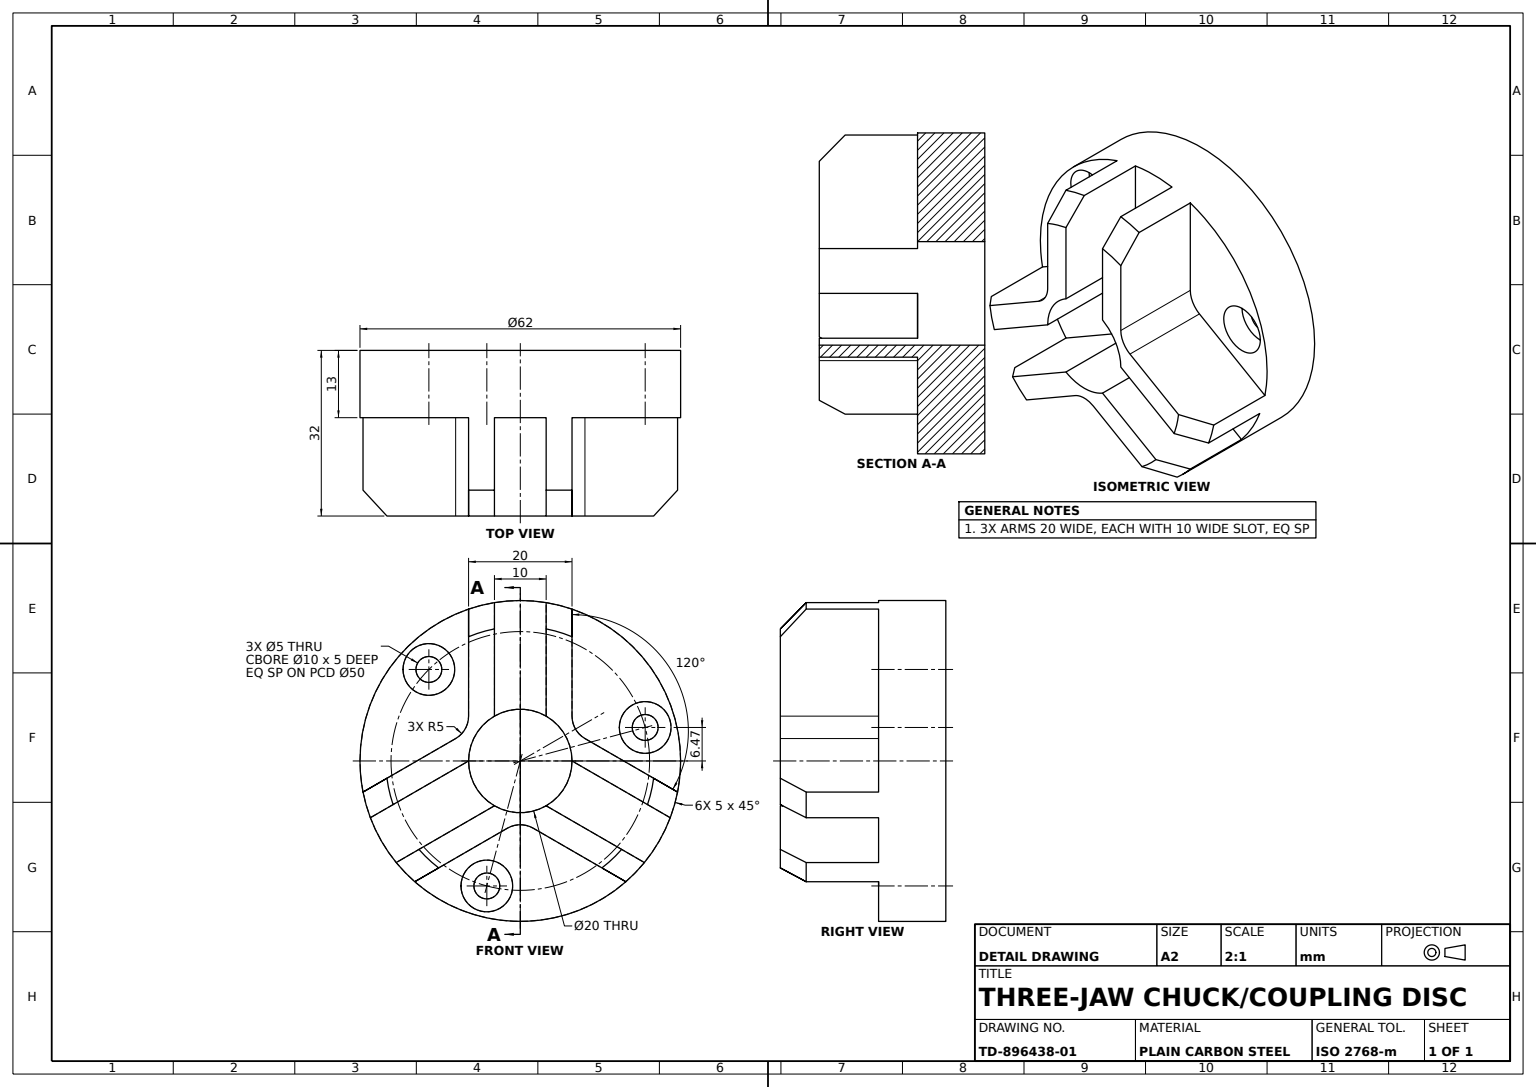
ISO-10303-21;
HEADER;
FILE_DESCRIPTION((''),'2;1');
FILE_NAME('','',(''),(''),'','','');
FILE_SCHEMA(('AUTOMOTIVE_DESIGN'));
ENDSEC;
DATA;
#1=APPLICATION_CONTEXT('');
#2=PRODUCT_CONTEXT('',#1,'mechanical');
#3=PRODUCT('','','',(#2));
#4=PRODUCT_DEFINITION_FORMATION('','',#3);
#5=PRODUCT_DEFINITION_CONTEXT('',#1,'design');
#6=PRODUCT_DEFINITION('','',#4,#5);
#7=PRODUCT_DEFINITION_SHAPE('','',#6);
#8=(LENGTH_UNIT()NAMED_UNIT(*)SI_UNIT(.MILLI.,.METRE.));
#9=(NAMED_UNIT(*)PLANE_ANGLE_UNIT()SI_UNIT($,.RADIAN.));
#10=(NAMED_UNIT(*)SI_UNIT($,.STERADIAN.)SOLID_ANGLE_UNIT());
#11=UNCERTAINTY_MEASURE_WITH_UNIT(LENGTH_MEASURE(1.E-05),#8,'distance_accuracy_value','');
#12=(GEOMETRIC_REPRESENTATION_CONTEXT(3)GLOBAL_UNCERTAINTY_ASSIGNED_CONTEXT((#11))GLOBAL_UNIT_ASSIGNED_CONTEXT((#8,#9,#10))REPRESENTATION_CONTEXT('',''));
#13=CARTESIAN_POINT('',(25.78461,-3.339746,32.));
#14=VERTEX_POINT('',#13);
#15=CARTESIAN_POINT('',(30.411612,-6.011147,27.));
#16=VERTEX_POINT('',#15);
#17=CARTESIAN_POINT('',(27.336826,-4.235919,30.345527));
#18=CARTESIAN_POINT('',(28.87747,-5.12541,28.676775));
#19=B_SPLINE_CURVE_WITH_KNOTS('',3,(#13,#17,#18,#15),.UNSPECIFIED.,.F.,.F.,(4,4),(0.,0.007317481),.UNSPECIFIED.);
#20=EDGE_CURVE('',#14,#16,#19,.T.);
#21=ORIENTED_EDGE('',*,*,#20,.T.);
#22=CARTESIAN_POINT('',(30.411612,-6.011147,13.));
#23=VERTEX_POINT('',#22);
#24=CARTESIAN_POINT('',(30.411612,-6.011147,32.));
#25=DIRECTION('',(0.,0.,-1.));
#26=VECTOR('',#25,1000.);
#27=LINE('',#24,#26);
#28=EDGE_CURVE('',#16,#23,#27,.T.);
#29=ORIENTED_EDGE('',*,*,#28,.T.);
#30=CARTESIAN_POINT('',(12.5,4.330127,13.));
#31=VERTEX_POINT('',#30);
#32=CARTESIAN_POINT('',(5.,8.660254,13.));
#33=DIRECTION('',(0.866025404,-0.5,0.));
#34=VECTOR('',#33,1000.);
#35=LINE('',#32,#34);
#36=EDGE_CURVE('',#31,#23,#35,.T.);
#37=ORIENTED_EDGE('',*,*,#36,.F.);
#38=CARTESIAN_POINT('',(12.5,4.330127,32.));
#39=VERTEX_POINT('',#38);
#40=LINE('',#38,#26);
#41=EDGE_CURVE('',#39,#31,#40,.T.);
#42=ORIENTED_EDGE('',*,*,#41,.F.);
#43=CARTESIAN_POINT('',(5.,8.660254,32.));
#44=LINE('',#43,#34);
#45=EDGE_CURVE('',#39,#14,#44,.T.);
#46=ORIENTED_EDGE('',*,*,#45,.T.);
#47=EDGE_LOOP('',(#21,#29,#37,#42,#46));
#48=FACE_OUTER_BOUND('',#47,.T.);
#49=DIRECTION('',(0.5,0.866025404,0.));
#50=DIRECTION('',(-0.866025404,0.5,0.));
#51=AXIS2_PLACEMENT_3D('',#43,#49,#50);
#52=PLANE('',#51);
#53=ADVANCED_FACE('',(#48),#52,.T.);
#54=CARTESIAN_POINT('',(-5.,-8.660254,32.));
#55=VERTEX_POINT('',#54);
#56=CARTESIAN_POINT('',(-5.,-8.660254,13.));
#57=VERTEX_POINT('',#56);
#58=LINE('',#54,#26);
#59=EDGE_CURVE('',#55,#57,#58,.T.);
#60=ORIENTED_EDGE('',*,*,#59,.F.);
#61=CARTESIAN_POINT('',(5.,-8.660254,32.));
#62=VERTEX_POINT('',#61);
#63=CARTESIAN_POINT('',(0.,0.,32.));
#64=DIRECTION('',(1.,0.,0.));
#65=AXIS2_PLACEMENT_3D('',#63,#25,#64);
#66=CIRCLE('',#65,10.);
#67=EDGE_CURVE('',#62,#55,#66,.T.);
#68=ORIENTED_EDGE('',*,*,#67,.F.);
#69=CARTESIAN_POINT('',(5.,-8.660254,13.));
#70=VERTEX_POINT('',#69);
#71=LINE('',#61,#26);
#72=EDGE_CURVE('',#62,#70,#71,.T.);
#73=ORIENTED_EDGE('',*,*,#72,.T.);
#74=CARTESIAN_POINT('',(10.,0.,13.));
#75=VERTEX_POINT('',#74);
#76=CARTESIAN_POINT('',(0.,0.,13.));
#77=DIRECTION('',(0.,0.,1.));
#78=AXIS2_PLACEMENT_3D('',#76,#77,#64);
#79=CIRCLE('',#78,10.);
#80=EDGE_CURVE('',#70,#75,#79,.T.);
#81=ORIENTED_EDGE('',*,*,#80,.T.);
#82=CARTESIAN_POINT('',(10.,0.,0.));
#83=VERTEX_POINT('',#82);
#84=VECTOR('',#77,1000.);
#85=LINE('',#82,#84);
#86=EDGE_CURVE('',#83,#75,#85,.T.);
#87=ORIENTED_EDGE('',*,*,#86,.F.);
#88=CARTESIAN_POINT('',(-10.,0.,0.));
#89=VERTEX_POINT('',#88);
#90=CARTESIAN_POINT('',(0.,0.,0.));
#91=AXIS2_PLACEMENT_3D('',#90,#77,#64);
#92=CIRCLE('',#91,10.);
#93=EDGE_CURVE('',#89,#83,#92,.T.);
#94=ORIENTED_EDGE('',*,*,#93,.F.);
#95=CARTESIAN_POINT('',(-10.,0.,13.));
#96=VERTEX_POINT('',#95);
#97=LINE('',#88,#84);
#98=EDGE_CURVE('',#89,#96,#97,.T.);
#99=ORIENTED_EDGE('',*,*,#98,.T.);
#100=EDGE_CURVE('',#96,#57,#79,.T.);
#101=ORIENTED_EDGE('',*,*,#100,.T.);
#102=EDGE_LOOP('',(#60,#68,#73,#81,#87,#94,#99,#101));
#103=FACE_OUTER_BOUND('',#102,.T.);
#104=CYLINDRICAL_SURFACE('',#91,10.);
#105=ADVANCED_FACE('',(#103),#104,.F.);
#106=CARTESIAN_POINT('',(-5.,8.660254,13.));
#107=VERTEX_POINT('',#106);
#108=CARTESIAN_POINT('',(-5.,30.594117,13.));
#109=VERTEX_POINT('',#108);
#110=CARTESIAN_POINT('',(-5.,0.,13.));
#111=DIRECTION('',(0.,1.,0.));
#112=VECTOR('',#111,1000.);
#113=LINE('',#110,#112);
#114=EDGE_CURVE('',#107,#109,#113,.T.);
#115=ORIENTED_EDGE('',*,*,#114,.T.);
#116=CARTESIAN_POINT('',(-5.,30.594117,27.));
#117=VERTEX_POINT('',#116);
#118=CARTESIAN_POINT('',(-5.,30.594117,32.));
#119=LINE('',#118,#26);
#120=EDGE_CURVE('',#117,#109,#119,.T.);
#121=ORIENTED_EDGE('',*,*,#120,.F.);
#122=CARTESIAN_POINT('',(-5.,25.514702,32.));
#123=VERTEX_POINT('',#122);
#124=CARTESIAN_POINT('',(-5.,28.903127,28.66885));
#125=CARTESIAN_POINT('',(-5.,27.210409,30.335943));
#126=B_SPLINE_CURVE_WITH_KNOTS('',3,(#116,#124,#125,#122),.UNSPECIFIED.,.F.,.F.,(4,4),(0.,0.007127444),.UNSPECIFIED.);
#127=EDGE_CURVE('',#117,#123,#126,.T.);
#128=ORIENTED_EDGE('',*,*,#127,.T.);
#129=CARTESIAN_POINT('',(-5.,8.660254,32.));
#130=VERTEX_POINT('',#129);
#131=CARTESIAN_POINT('',(-5.,0.,32.));
#132=LINE('',#131,#112);
#133=EDGE_CURVE('',#130,#123,#132,.T.);
#134=ORIENTED_EDGE('',*,*,#133,.F.);
#135=LINE('',#129,#26);
#136=EDGE_CURVE('',#130,#107,#135,.T.);
#137=ORIENTED_EDGE('',*,*,#136,.T.);
#138=EDGE_LOOP('',(#115,#121,#128,#134,#137));
#139=FACE_OUTER_BOUND('',#138,.T.);
#140=DIRECTION('',(-1.,0.,0.));
#141=AXIS2_PLACEMENT_3D('',#131,#140,#77);
#142=PLANE('',#141);
#143=ADVANCED_FACE('',(#139),#142,.F.);
#144=CARTESIAN_POINT('',(5.,30.594117,13.));
#145=VERTEX_POINT('',#144);
#146=CIRCLE('',#78,31.);
#147=EDGE_CURVE('',#145,#109,#146,.T.);
#148=ORIENTED_EDGE('',*,*,#147,.T.);
#149=ORIENTED_EDGE('',*,*,#114,.F.);
#150=VERTEX_POINT('',#32);
#151=EDGE_CURVE('',#150,#107,#79,.T.);
#152=ORIENTED_EDGE('',*,*,#151,.F.);
#153=CARTESIAN_POINT('',(5.,0.,13.));
#154=LINE('',#153,#112);
#155=EDGE_CURVE('',#150,#145,#154,.T.);
#156=ORIENTED_EDGE('',*,*,#155,.T.);
#157=EDGE_LOOP('',(#148,#149,#152,#156));
#158=FACE_OUTER_BOUND('',#157,.T.);
#159=PLANE('',#78);
#160=ADVANCED_FACE('',(#158),#159,.T.);
#161=CARTESIAN_POINT('',(-28.995283,-10.966932,13.));
#162=VERTEX_POINT('',#161);
#163=CARTESIAN_POINT('',(-2.5,4.330127,13.));
#164=DIRECTION('',(-0.866025404,-0.5,0.));
#165=VECTOR('',#164,1000.);
#166=LINE('',#163,#165);
#167=EDGE_CURVE('',#96,#162,#166,.T.);
#168=ORIENTED_EDGE('',*,*,#167,.T.);
#169=CARTESIAN_POINT('',(-23.995283,-19.627186,13.));
#170=VERTEX_POINT('',#169);
#171=EDGE_CURVE('',#162,#170,#146,.T.);
#172=ORIENTED_EDGE('',*,*,#171,.T.);
#173=CARTESIAN_POINT('',(2.5,-4.330127,13.));
#174=LINE('',#173,#165);
#175=EDGE_CURVE('',#57,#170,#174,.T.);
#176=ORIENTED_EDGE('',*,*,#175,.F.);
#177=ORIENTED_EDGE('',*,*,#100,.F.);
#178=EDGE_LOOP('',(#168,#172,#176,#177));
#179=FACE_OUTER_BOUND('',#178,.T.);
#180=ADVANCED_FACE('',(#179),#159,.T.);
#181=CARTESIAN_POINT('',(-1.470476,-24.148146,13.));
#182=VERTEX_POINT('',#181);
#183=CARTESIAN_POINT('',(-11.470476,-24.148146,13.));
#184=VERTEX_POINT('',#183);
#185=CARTESIAN_POINT('',(-6.470476,-24.148146,13.));
#186=AXIS2_PLACEMENT_3D('',#185,#77,#64);
#187=CIRCLE('',#186,5.);
#188=EDGE_CURVE('',#182,#184,#187,.T.);
#189=ORIENTED_EDGE('',*,*,#188,.F.);
#190=EDGE_CURVE('',#184,#182,#187,.T.);
#191=ORIENTED_EDGE('',*,*,#190,.F.);
#192=EDGE_LOOP('',(#189,#191));
#193=FACE_BOUND('',#192,.T.);
#194=CARTESIAN_POINT('',(2.5,-12.990381,13.));
#195=VERTEX_POINT('',#194);
#196=CARTESIAN_POINT('',(-2.5,-12.990381,13.));
#197=VERTEX_POINT('',#196);
#198=CARTESIAN_POINT('',(0.,-17.320508,13.));
#199=AXIS2_PLACEMENT_3D('',#198,#77,#64);
#200=CIRCLE('',#199,5.);
#201=EDGE_CURVE('',#195,#197,#200,.T.);
#202=ORIENTED_EDGE('',*,*,#201,.T.);
#203=CARTESIAN_POINT('',(-20.411612,-23.331655,13.));
#204=VERTEX_POINT('',#203);
#205=LINE('',#69,#165);
#206=EDGE_CURVE('',#197,#204,#205,.T.);
#207=ORIENTED_EDGE('',*,*,#206,.T.);
#208=CARTESIAN_POINT('',(20.411612,-23.331655,13.));
#209=VERTEX_POINT('',#208);
#210=EDGE_CURVE('',#204,#209,#146,.T.);
#211=ORIENTED_EDGE('',*,*,#210,.T.);
#212=LINE('',#56,#34);
#213=EDGE_CURVE('',#195,#209,#212,.T.);
#214=ORIENTED_EDGE('',*,*,#213,.F.);
#215=EDGE_LOOP('',(#202,#207,#211,#214));
#216=FACE_OUTER_BOUND('',#215,.T.);
#217=ADVANCED_FACE('',(#193,#216),#159,.T.);
#218=CARTESIAN_POINT('',(26.648146,6.470476,0.));
#219=VERTEX_POINT('',#218);
#220=CARTESIAN_POINT('',(26.648146,6.470476,8.));
#221=VERTEX_POINT('',#220);
#222=LINE('',#218,#84);
#223=EDGE_CURVE('',#219,#221,#222,.T.);
#224=ORIENTED_EDGE('',*,*,#223,.T.);
#225=CARTESIAN_POINT('',(21.648146,6.470476,8.));
#226=VERTEX_POINT('',#225);
#227=CARTESIAN_POINT('',(24.148146,6.470476,8.));
#228=AXIS2_PLACEMENT_3D('',#227,#25,#64);
#229=CIRCLE('',#228,2.5);
#230=EDGE_CURVE('',#226,#221,#229,.T.);
#231=ORIENTED_EDGE('',*,*,#230,.F.);
#232=CARTESIAN_POINT('',(21.648146,6.470476,0.));
#233=VERTEX_POINT('',#232);
#234=LINE('',#232,#84);
#235=EDGE_CURVE('',#233,#226,#234,.T.);
#236=ORIENTED_EDGE('',*,*,#235,.F.);
#237=CARTESIAN_POINT('',(24.148146,6.470476,0.));
#238=DIRECTION('',(-0.5,0.866025404,0.));
#239=AXIS2_PLACEMENT_3D('',#237,#77,#238);
#240=CIRCLE('',#239,2.5);
#241=EDGE_CURVE('',#219,#233,#240,.T.);
#242=ORIENTED_EDGE('',*,*,#241,.F.);
#243=EDGE_LOOP('',(#224,#231,#236,#242));
#244=FACE_OUTER_BOUND('',#243,.T.);
#245=AXIS2_PLACEMENT_3D('',#237,#77,#64);
#246=CYLINDRICAL_SURFACE('',#245,2.5);
#247=ADVANCED_FACE('',(#244),#246,.F.);
#248=ORIENTED_EDGE('',*,*,#20,.F.);
#249=CARTESIAN_POINT('',(24.59638,-8.427224,32.));
#250=VERTEX_POINT('',#249);
#251=AXIS2_PLACEMENT_3D('',#63,#77,#64);
#252=CIRCLE('',#251,26.);
#253=EDGE_CURVE('',#250,#14,#252,.T.);
#254=ORIENTED_EDGE('',*,*,#253,.F.);
#255=CARTESIAN_POINT('',(28.995283,-10.966932,27.));
#256=VERTEX_POINT('',#255);
#257=CARTESIAN_POINT('',(27.530843,-10.121437,28.66885));
#258=CARTESIAN_POINT('',(26.064906,-9.275078,30.335943));
#259=B_SPLINE_CURVE_WITH_KNOTS('',3,(#255,#257,#258,#249),.UNSPECIFIED.,.F.,.F.,(4,4),(0.,0.007127444),.UNSPECIFIED.);
#260=EDGE_CURVE('',#256,#250,#259,.T.);
#261=ORIENTED_EDGE('',*,*,#260,.F.);
#262=CARTESIAN_POINT('',(0.,0.,27.));
#263=AXIS2_PLACEMENT_3D('',#262,#25,#64);
#264=CIRCLE('',#263,31.);
#265=EDGE_CURVE('',#16,#256,#264,.T.);
#266=ORIENTED_EDGE('',*,*,#265,.F.);
#267=EDGE_LOOP('',(#248,#254,#261,#266));
#268=FACE_OUTER_BOUND('',#267,.T.);
#269=AXIS2_PLACEMENT_3D('',#63,#25,#140);
#270=CONICAL_SURFACE('',#269,26.,0.785398163);
#271=ADVANCED_FACE('',(#268),#270,.T.);
#272=CARTESIAN_POINT('',(10.,29.342802,27.));
#273=VERTEX_POINT('',#272);
#274=CARTESIAN_POINT('',(10.,29.342802,13.));
#275=VERTEX_POINT('',#274);
#276=CARTESIAN_POINT('',(10.,29.342802,32.));
#277=LINE('',#276,#26);
#278=EDGE_CURVE('',#273,#275,#277,.T.);
#279=ORIENTED_EDGE('',*,*,#278,.F.);
#280=CARTESIAN_POINT('',(10.,24.,32.));
#281=VERTEX_POINT('',#280);
#282=CARTESIAN_POINT('',(10.,27.571327,28.676775));
#283=CARTESIAN_POINT('',(10.,25.792345,30.345527));
#284=B_SPLINE_CURVE_WITH_KNOTS('',3,(#272,#282,#283,#280),.UNSPECIFIED.,.F.,.F.,(4,4),(0.,0.007317481),.UNSPECIFIED.);
#285=EDGE_CURVE('',#273,#281,#284,.T.);
#286=ORIENTED_EDGE('',*,*,#285,.T.);
#287=CARTESIAN_POINT('',(10.,8.660254,32.));
#288=VERTEX_POINT('',#287);
#289=CARTESIAN_POINT('',(10.,0.,32.));
#290=LINE('',#289,#112);
#291=EDGE_CURVE('',#288,#281,#290,.T.);
#292=ORIENTED_EDGE('',*,*,#291,.F.);
#293=CARTESIAN_POINT('',(10.,8.660254,13.));
#294=VERTEX_POINT('',#293);
#295=LINE('',#287,#26);
#296=EDGE_CURVE('',#288,#294,#295,.T.);
#297=ORIENTED_EDGE('',*,*,#296,.T.);
#298=LINE('',#74,#112);
#299=EDGE_CURVE('',#294,#275,#298,.T.);
#300=ORIENTED_EDGE('',*,*,#299,.T.);
#301=EDGE_LOOP('',(#279,#286,#292,#297,#300));
#302=FACE_OUTER_BOUND('',#301,.T.);
#303=AXIS2_PLACEMENT_3D('',#289,#140,#77);
#304=PLANE('',#303);
#305=ADVANCED_FACE('',(#302),#304,.F.);
#306=CARTESIAN_POINT('',(-19.59638,-17.087478,32.));
#307=VERTEX_POINT('',#306);
#308=CARTESIAN_POINT('',(-15.78461,-20.660254,32.));
#309=VERTEX_POINT('',#308);
#310=EDGE_CURVE('',#307,#309,#252,.T.);
#311=ORIENTED_EDGE('',*,*,#310,.T.);
#312=CARTESIAN_POINT('',(-2.5,-12.990381,32.));
#313=VERTEX_POINT('',#312);
#314=LINE('',#61,#165);
#315=EDGE_CURVE('',#313,#309,#314,.T.);
#316=ORIENTED_EDGE('',*,*,#315,.F.);
#317=CARTESIAN_POINT('',(2.5,-12.990381,32.));
#318=VERTEX_POINT('',#317);
#319=CARTESIAN_POINT('',(0.,-17.320508,32.));
#320=AXIS2_PLACEMENT_3D('',#319,#77,#64);
#321=CIRCLE('',#320,5.);
#322=EDGE_CURVE('',#318,#313,#321,.T.);
#323=ORIENTED_EDGE('',*,*,#322,.F.);
#324=CARTESIAN_POINT('',(15.78461,-20.660254,32.));
#325=VERTEX_POINT('',#324);
#326=LINE('',#54,#34);
#327=EDGE_CURVE('',#318,#325,#326,.T.);
#328=ORIENTED_EDGE('',*,*,#327,.T.);
#329=CARTESIAN_POINT('',(19.59638,-17.087478,32.));
#330=VERTEX_POINT('',#329);
#331=EDGE_CURVE('',#325,#330,#252,.T.);
#332=ORIENTED_EDGE('',*,*,#331,.T.);
#333=CARTESIAN_POINT('',(-2.5,-4.330127,32.));
#334=LINE('',#333,#34);
#335=EDGE_CURVE('',#62,#330,#334,.T.);
#336=ORIENTED_EDGE('',*,*,#335,.F.);
#337=ORIENTED_EDGE('',*,*,#67,.T.);
#338=CARTESIAN_POINT('',(2.5,-4.330127,32.));
#339=LINE('',#338,#165);
#340=EDGE_CURVE('',#55,#307,#339,.T.);
#341=ORIENTED_EDGE('',*,*,#340,.T.);
#342=EDGE_LOOP('',(#311,#316,#323,#328,#332,#336,#337,#341));
#343=FACE_OUTER_BOUND('',#342,.T.);
#344=PLANE('',#251);
#345=ADVANCED_FACE('',(#343),#344,.T.);
#346=CARTESIAN_POINT('',(-8.970476,-24.148146,0.));
#347=VERTEX_POINT('',#346);
#348=CARTESIAN_POINT('',(-3.970476,-24.148146,0.));
#349=VERTEX_POINT('',#348);
#350=CARTESIAN_POINT('',(-6.470476,-24.148146,0.));
#351=AXIS2_PLACEMENT_3D('',#350,#77,#64);
#352=CIRCLE('',#351,2.5);
#353=EDGE_CURVE('',#347,#349,#352,.T.);
#354=ORIENTED_EDGE('',*,*,#353,.F.);
#355=CARTESIAN_POINT('',(-8.970476,-24.148146,8.));
#356=VERTEX_POINT('',#355);
#357=LINE('',#346,#84);
#358=EDGE_CURVE('',#347,#356,#357,.T.);
#359=ORIENTED_EDGE('',*,*,#358,.T.);
#360=CARTESIAN_POINT('',(-3.970476,-24.148146,8.));
#361=VERTEX_POINT('',#360);
#362=CARTESIAN_POINT('',(-6.470476,-24.148146,8.));
#363=AXIS2_PLACEMENT_3D('',#362,#25,#64);
#364=CIRCLE('',#363,2.5);
#365=EDGE_CURVE('',#361,#356,#364,.T.);
#366=ORIENTED_EDGE('',*,*,#365,.F.);
#367=LINE('',#348,#84);
#368=EDGE_CURVE('',#349,#361,#367,.T.);
#369=ORIENTED_EDGE('',*,*,#368,.F.);
#370=EDGE_LOOP('',(#354,#359,#366,#369));
#371=FACE_OUTER_BOUND('',#370,.T.);
#372=CYLINDRICAL_SURFACE('',#351,2.5);
#373=ADVANCED_FACE('',(#371),#372,.F.);
#374=CARTESIAN_POINT('',(23.995283,-19.627186,27.));
#375=VERTEX_POINT('',#374);
#376=CARTESIAN_POINT('',(20.411612,-23.331655,27.));
#377=VERTEX_POINT('',#376);
#378=EDGE_CURVE('',#375,#377,#264,.T.);
#379=ORIENTED_EDGE('',*,*,#378,.F.);
#380=CARTESIAN_POINT('',(21.064906,-17.935332,30.335943));
#381=CARTESIAN_POINT('',(22.530843,-18.781691,28.66885));
#382=B_SPLINE_CURVE_WITH_KNOTS('',3,(#329,#380,#381,#374),.UNSPECIFIED.,.F.,.F.,(4,4),(0.,0.007127444),.UNSPECIFIED.);
#383=EDGE_CURVE('',#330,#375,#382,.T.);
#384=ORIENTED_EDGE('',*,*,#383,.F.);
#385=ORIENTED_EDGE('',*,*,#331,.F.);
#386=CARTESIAN_POINT('',(18.87747,-22.445918,28.676775));
#387=CARTESIAN_POINT('',(17.336826,-21.556427,30.345527));
#388=B_SPLINE_CURVE_WITH_KNOTS('',3,(#376,#386,#387,#324),.UNSPECIFIED.,.F.,.F.,(4,4),(0.,0.007317481),.UNSPECIFIED.);
#389=EDGE_CURVE('',#377,#325,#388,.T.);
#390=ORIENTED_EDGE('',*,*,#389,.F.);
#391=EDGE_LOOP('',(#379,#384,#385,#390));
#392=FACE_OUTER_BOUND('',#391,.T.);
#393=ADVANCED_FACE('',(#392),#270,.T.);
#394=ORIENTED_EDGE('',*,*,#253,.T.);
#395=ORIENTED_EDGE('',*,*,#45,.F.);
#396=CARTESIAN_POINT('',(15.,8.660254,32.));
#397=AXIS2_PLACEMENT_3D('',#396,#77,#64);
#398=CIRCLE('',#397,5.);
#399=EDGE_CURVE('',#288,#39,#398,.T.);
#400=ORIENTED_EDGE('',*,*,#399,.F.);
#401=ORIENTED_EDGE('',*,*,#291,.T.);
#402=CARTESIAN_POINT('',(5.,25.514702,32.));
#403=VERTEX_POINT('',#402);
#404=EDGE_CURVE('',#281,#403,#252,.T.);
#405=ORIENTED_EDGE('',*,*,#404,.T.);
#406=VERTEX_POINT('',#43);
#407=CARTESIAN_POINT('',(5.,0.,32.));
#408=LINE('',#407,#112);
#409=EDGE_CURVE('',#406,#403,#408,.T.);
#410=ORIENTED_EDGE('',*,*,#409,.F.);
#411=VERTEX_POINT('',#289);
#412=EDGE_CURVE('',#406,#411,#66,.T.);
#413=ORIENTED_EDGE('',*,*,#412,.T.);
#414=CARTESIAN_POINT('',(2.5,4.330127,32.));
#415=LINE('',#414,#34);
#416=EDGE_CURVE('',#411,#250,#415,.T.);
#417=ORIENTED_EDGE('',*,*,#416,.T.);
#418=EDGE_LOOP('',(#394,#395,#400,#401,#405,#410,#413,#417));
#419=FACE_OUTER_BOUND('',#418,.T.);
#420=ADVANCED_FACE('',(#419),#344,.T.);
#421=CARTESIAN_POINT('',(19.148146,6.470476,8.));
#422=VERTEX_POINT('',#421);
#423=CARTESIAN_POINT('',(29.148146,6.470476,8.));
#424=VERTEX_POINT('',#423);
#425=AXIS2_PLACEMENT_3D('',#227,#77,#238);
#426=CIRCLE('',#425,5.);
#427=EDGE_CURVE('',#422,#424,#426,.T.);
#428=ORIENTED_EDGE('',*,*,#427,.F.);
#429=CARTESIAN_POINT('',(19.148146,6.470476,13.));
#430=VERTEX_POINT('',#429);
#431=LINE('',#421,#84);
#432=EDGE_CURVE('',#422,#430,#431,.T.);
#433=ORIENTED_EDGE('',*,*,#432,.T.);
#434=CARTESIAN_POINT('',(29.148146,6.470476,13.));
#435=VERTEX_POINT('',#434);
#436=CARTESIAN_POINT('',(24.148146,6.470476,13.));
#437=AXIS2_PLACEMENT_3D('',#436,#77,#238);
#438=CIRCLE('',#437,5.);
#439=EDGE_CURVE('',#430,#435,#438,.T.);
#440=ORIENTED_EDGE('',*,*,#439,.T.);
#441=LINE('',#423,#84);
#442=EDGE_CURVE('',#424,#435,#441,.T.);
#443=ORIENTED_EDGE('',*,*,#442,.F.);
#444=EDGE_LOOP('',(#428,#433,#440,#443));
#445=FACE_OUTER_BOUND('',#444,.T.);
#446=AXIS2_PLACEMENT_3D('',#227,#77,#64);
#447=CYLINDRICAL_SURFACE('',#446,5.);
#448=ADVANCED_FACE('',(#445),#447,.F.);
#449=CARTESIAN_POINT('',(20.411612,-23.331655,32.));
#450=LINE('',#449,#26);
#451=EDGE_CURVE('',#377,#209,#450,.T.);
#452=ORIENTED_EDGE('',*,*,#451,.F.);
#453=ORIENTED_EDGE('',*,*,#389,.T.);
#454=ORIENTED_EDGE('',*,*,#327,.F.);
#455=LINE('',#317,#26);
#456=EDGE_CURVE('',#318,#195,#455,.T.);
#457=ORIENTED_EDGE('',*,*,#456,.T.);
#458=ORIENTED_EDGE('',*,*,#213,.T.);
#459=EDGE_LOOP('',(#452,#453,#454,#457,#458));
#460=FACE_OUTER_BOUND('',#459,.T.);
#461=AXIS2_PLACEMENT_3D('',#54,#49,#50);
#462=PLANE('',#461);
#463=ADVANCED_FACE('',(#460),#462,.F.);
#464=ORIENTED_EDGE('',*,*,#136,.F.);
#465=CARTESIAN_POINT('',(-10.,0.,32.));
#466=VERTEX_POINT('',#465);
#467=EDGE_CURVE('',#466,#130,#66,.T.);
#468=ORIENTED_EDGE('',*,*,#467,.F.);
#469=LINE('',#465,#26);
#470=EDGE_CURVE('',#466,#96,#469,.T.);
#471=ORIENTED_EDGE('',*,*,#470,.T.);
#472=ORIENTED_EDGE('',*,*,#98,.F.);
#473=EDGE_CURVE('',#83,#89,#92,.T.);
#474=ORIENTED_EDGE('',*,*,#473,.F.);
#475=ORIENTED_EDGE('',*,*,#86,.T.);
#476=LINE('',#289,#26);
#477=EDGE_CURVE('',#411,#75,#476,.T.);
#478=ORIENTED_EDGE('',*,*,#477,.F.);
#479=ORIENTED_EDGE('',*,*,#412,.F.);
#480=LINE('',#43,#26);
#481=EDGE_CURVE('',#406,#150,#480,.T.);
#482=ORIENTED_EDGE('',*,*,#481,.T.);
#483=ORIENTED_EDGE('',*,*,#151,.T.);
#484=EDGE_LOOP('',(#464,#468,#471,#472,#474,#475,#478,#479,#482,#483));
#485=FACE_OUTER_BOUND('',#484,.T.);
#486=ADVANCED_FACE('',(#485),#104,.F.);
#487=EDGE_CURVE('',#435,#430,#438,.T.);
#488=ORIENTED_EDGE('',*,*,#487,.T.);
#489=ORIENTED_EDGE('',*,*,#432,.F.);
#490=EDGE_CURVE('',#424,#422,#426,.T.);
#491=ORIENTED_EDGE('',*,*,#490,.F.);
#492=ORIENTED_EDGE('',*,*,#442,.T.);
#493=EDGE_LOOP('',(#488,#489,#491,#492));
#494=FACE_OUTER_BOUND('',#493,.T.);
#495=ADVANCED_FACE('',(#494),#447,.F.);
#496=ORIENTED_EDGE('',*,*,#285,.F.);
#497=CARTESIAN_POINT('',(5.,30.594117,27.));
#498=VERTEX_POINT('',#497);
#499=EDGE_CURVE('',#498,#273,#264,.T.);
#500=ORIENTED_EDGE('',*,*,#499,.F.);
#501=CARTESIAN_POINT('',(5.,27.210409,30.335943));
#502=CARTESIAN_POINT('',(5.,28.903127,28.66885));
#503=B_SPLINE_CURVE_WITH_KNOTS('',3,(#402,#501,#502,#497),.UNSPECIFIED.,.F.,.F.,(4,4),(0.,0.007127444),.UNSPECIFIED.);
#504=EDGE_CURVE('',#403,#498,#503,.T.);
#505=ORIENTED_EDGE('',*,*,#504,.F.);
#506=ORIENTED_EDGE('',*,*,#404,.F.);
#507=EDGE_LOOP('',(#496,#500,#505,#506));
#508=FACE_OUTER_BOUND('',#507,.T.);
#509=ADVANCED_FACE('',(#508),#270,.T.);
#510=CARTESIAN_POINT('',(-12.5,4.330127,32.));
#511=VERTEX_POINT('',#510);
#512=CARTESIAN_POINT('',(-25.78461,-3.339746,32.));
#513=VERTEX_POINT('',#512);
#514=LINE('',#129,#165);
#515=EDGE_CURVE('',#511,#513,#514,.T.);
#516=ORIENTED_EDGE('',*,*,#515,.T.);
#517=CARTESIAN_POINT('',(-24.59638,-8.427224,32.));
#518=VERTEX_POINT('',#517);
#519=EDGE_CURVE('',#513,#518,#252,.T.);
#520=ORIENTED_EDGE('',*,*,#519,.T.);
#521=CARTESIAN_POINT('',(-2.5,4.330127,32.));
#522=LINE('',#521,#165);
#523=EDGE_CURVE('',#466,#518,#522,.T.);
#524=ORIENTED_EDGE('',*,*,#523,.F.);
#525=ORIENTED_EDGE('',*,*,#467,.T.);
#526=ORIENTED_EDGE('',*,*,#133,.T.);
#527=CARTESIAN_POINT('',(-10.,24.,32.));
#528=VERTEX_POINT('',#527);
#529=EDGE_CURVE('',#123,#528,#252,.T.);
#530=ORIENTED_EDGE('',*,*,#529,.T.);
#531=CARTESIAN_POINT('',(-10.,8.660254,32.));
#532=VERTEX_POINT('',#531);
#533=LINE('',#465,#112);
#534=EDGE_CURVE('',#532,#528,#533,.T.);
#535=ORIENTED_EDGE('',*,*,#534,.F.);
#536=CARTESIAN_POINT('',(-15.,8.660254,32.));
#537=AXIS2_PLACEMENT_3D('',#536,#77,#64);
#538=CIRCLE('',#537,5.);
#539=EDGE_CURVE('',#511,#532,#538,.T.);
#540=ORIENTED_EDGE('',*,*,#539,.F.);
#541=EDGE_LOOP('',(#516,#520,#524,#525,#526,#530,#535,#540));
#542=FACE_OUTER_BOUND('',#541,.T.);
#543=ADVANCED_FACE('',(#542),#344,.T.);
#544=ORIENTED_EDGE('',*,*,#155,.F.);
#545=ORIENTED_EDGE('',*,*,#481,.F.);
#546=ORIENTED_EDGE('',*,*,#409,.T.);
#547=ORIENTED_EDGE('',*,*,#504,.T.);
#548=CARTESIAN_POINT('',(5.,30.594117,32.));
#549=LINE('',#548,#26);
#550=EDGE_CURVE('',#498,#145,#549,.T.);
#551=ORIENTED_EDGE('',*,*,#550,.T.);
#552=EDGE_LOOP('',(#544,#545,#546,#547,#551));
#553=FACE_OUTER_BOUND('',#552,.T.);
#554=AXIS2_PLACEMENT_3D('',#407,#140,#77);
#555=PLANE('',#554);
#556=ADVANCED_FACE('',(#553),#555,.T.);
#557=CARTESIAN_POINT('',(-22.67767,17.67767,13.));
#558=VERTEX_POINT('',#557);
#559=CARTESIAN_POINT('',(-12.67767,17.67767,13.));
#560=VERTEX_POINT('',#559);
#561=CARTESIAN_POINT('',(-17.67767,17.67767,13.));
#562=DIRECTION('',(-0.5,-0.866025404,0.));
#563=AXIS2_PLACEMENT_3D('',#561,#77,#562);
#564=CIRCLE('',#563,5.);
#565=EDGE_CURVE('',#558,#560,#564,.T.);
#566=ORIENTED_EDGE('',*,*,#565,.F.);
#567=EDGE_CURVE('',#560,#558,#564,.T.);
#568=ORIENTED_EDGE('',*,*,#567,.F.);
#569=EDGE_LOOP('',(#566,#568));
#570=FACE_BOUND('',#569,.T.);
#571=CARTESIAN_POINT('',(-10.,29.342802,13.));
#572=VERTEX_POINT('',#571);
#573=CARTESIAN_POINT('',(-31.,0.,13.));
#574=VERTEX_POINT('',#573);
#575=EDGE_CURVE('',#572,#574,#146,.T.);
#576=ORIENTED_EDGE('',*,*,#575,.T.);
#577=CARTESIAN_POINT('',(-30.411612,-6.011147,13.));
#578=VERTEX_POINT('',#577);
#579=EDGE_CURVE('',#574,#578,#146,.T.);
#580=ORIENTED_EDGE('',*,*,#579,.T.);
#581=CARTESIAN_POINT('',(-12.5,4.330127,13.));
#582=VERTEX_POINT('',#581);
#583=LINE('',#106,#165);
#584=EDGE_CURVE('',#582,#578,#583,.T.);
#585=ORIENTED_EDGE('',*,*,#584,.F.);
#586=CARTESIAN_POINT('',(-10.,8.660254,13.));
#587=VERTEX_POINT('',#586);
#588=CARTESIAN_POINT('',(-15.,8.660254,13.));
#589=AXIS2_PLACEMENT_3D('',#588,#77,#64);
#590=CIRCLE('',#589,5.);
#591=EDGE_CURVE('',#582,#587,#590,.T.);
#592=ORIENTED_EDGE('',*,*,#591,.T.);
#593=LINE('',#95,#112);
#594=EDGE_CURVE('',#587,#572,#593,.T.);
#595=ORIENTED_EDGE('',*,*,#594,.T.);
#596=EDGE_LOOP('',(#576,#580,#585,#592,#595));
#597=FACE_OUTER_BOUND('',#596,.T.);
#598=ADVANCED_FACE('',(#570,#597),#159,.T.);
#599=ORIENTED_EDGE('',*,*,#565,.T.);
#600=CARTESIAN_POINT('',(-12.67767,17.67767,8.));
#601=VERTEX_POINT('',#600);
#602=LINE('',#600,#84);
#603=EDGE_CURVE('',#601,#560,#602,.T.);
#604=ORIENTED_EDGE('',*,*,#603,.F.);
#605=CARTESIAN_POINT('',(-22.67767,17.67767,8.));
#606=VERTEX_POINT('',#605);
#607=CARTESIAN_POINT('',(-17.67767,17.67767,8.));
#608=AXIS2_PLACEMENT_3D('',#607,#77,#562);
#609=CIRCLE('',#608,5.);
#610=EDGE_CURVE('',#606,#601,#609,.T.);
#611=ORIENTED_EDGE('',*,*,#610,.F.);
#612=LINE('',#605,#84);
#613=EDGE_CURVE('',#606,#558,#612,.T.);
#614=ORIENTED_EDGE('',*,*,#613,.T.);
#615=EDGE_LOOP('',(#599,#604,#611,#614));
#616=FACE_OUTER_BOUND('',#615,.T.);
#617=AXIS2_PLACEMENT_3D('',#607,#77,#64);
#618=CYLINDRICAL_SURFACE('',#617,5.);
#619=ADVANCED_FACE('',(#616),#618,.F.);
#620=CARTESIAN_POINT('',(28.995283,-10.966932,13.));
#621=VERTEX_POINT('',#620);
#622=CARTESIAN_POINT('',(28.995283,-10.966932,32.));
#623=LINE('',#622,#26);
#624=EDGE_CURVE('',#256,#621,#623,.T.);
#625=ORIENTED_EDGE('',*,*,#624,.F.);
#626=ORIENTED_EDGE('',*,*,#260,.T.);
#627=ORIENTED_EDGE('',*,*,#416,.F.);
#628=ORIENTED_EDGE('',*,*,#477,.T.);
#629=CARTESIAN_POINT('',(2.5,4.330127,13.));
#630=LINE('',#629,#34);
#631=EDGE_CURVE('',#75,#621,#630,.T.);
#632=ORIENTED_EDGE('',*,*,#631,.T.);
#633=EDGE_LOOP('',(#625,#626,#627,#628,#632));
#634=FACE_OUTER_BOUND('',#633,.T.);
#635=AXIS2_PLACEMENT_3D('',#414,#49,#50);
#636=PLANE('',#635);
#637=ADVANCED_FACE('',(#634),#636,.F.);
#638=CARTESIAN_POINT('',(-15.17767,17.67767,8.));
#639=VERTEX_POINT('',#638);
#640=CARTESIAN_POINT('',(-20.17767,17.67767,8.));
#641=VERTEX_POINT('',#640);
#642=AXIS2_PLACEMENT_3D('',#607,#25,#64);
#643=CIRCLE('',#642,2.5);
#644=EDGE_CURVE('',#639,#641,#643,.T.);
#645=ORIENTED_EDGE('',*,*,#644,.F.);
#646=CARTESIAN_POINT('',(-15.17767,17.67767,0.));
#647=VERTEX_POINT('',#646);
#648=LINE('',#646,#84);
#649=EDGE_CURVE('',#647,#639,#648,.T.);
#650=ORIENTED_EDGE('',*,*,#649,.F.);
#651=CARTESIAN_POINT('',(-20.17767,17.67767,0.));
#652=VERTEX_POINT('',#651);
#653=CARTESIAN_POINT('',(-17.67767,17.67767,0.));
#654=AXIS2_PLACEMENT_3D('',#653,#77,#562);
#655=CIRCLE('',#654,2.5);
#656=EDGE_CURVE('',#652,#647,#655,.T.);
#657=ORIENTED_EDGE('',*,*,#656,.F.);
#658=LINE('',#651,#84);
#659=EDGE_CURVE('',#652,#641,#658,.T.);
#660=ORIENTED_EDGE('',*,*,#659,.T.);
#661=EDGE_LOOP('',(#645,#650,#657,#660));
#662=FACE_OUTER_BOUND('',#661,.T.);
#663=AXIS2_PLACEMENT_3D('',#653,#77,#64);
#664=CYLINDRICAL_SURFACE('',#663,2.5);
#665=ADVANCED_FACE('',(#662),#664,.F.);
#666=CARTESIAN_POINT('',(-1.470476,-24.148146,8.));
#667=VERTEX_POINT('',#666);
#668=CARTESIAN_POINT('',(-11.470476,-24.148146,8.));
#669=VERTEX_POINT('',#668);
#670=AXIS2_PLACEMENT_3D('',#362,#77,#64);
#671=CIRCLE('',#670,5.);
#672=EDGE_CURVE('',#667,#669,#671,.T.);
#673=ORIENTED_EDGE('',*,*,#672,.F.);
#674=LINE('',#666,#84);
#675=EDGE_CURVE('',#667,#182,#674,.T.);
#676=ORIENTED_EDGE('',*,*,#675,.T.);
#677=ORIENTED_EDGE('',*,*,#188,.T.);
#678=LINE('',#668,#84);
#679=EDGE_CURVE('',#669,#184,#678,.T.);
#680=ORIENTED_EDGE('',*,*,#679,.F.);
#681=EDGE_LOOP('',(#673,#676,#677,#680));
#682=FACE_OUTER_BOUND('',#681,.T.);
#683=CYLINDRICAL_SURFACE('',#670,5.);
#684=ADVANCED_FACE('',(#682),#683,.F.);
#685=ORIENTED_EDGE('',*,*,#80,.F.);
#686=CARTESIAN_POINT('',(23.995283,-19.627186,13.));
#687=VERTEX_POINT('',#686);
#688=CARTESIAN_POINT('',(-2.5,-4.330127,13.));
#689=LINE('',#688,#34);
#690=EDGE_CURVE('',#70,#687,#689,.T.);
#691=ORIENTED_EDGE('',*,*,#690,.T.);
#692=EDGE_CURVE('',#687,#621,#146,.T.);
#693=ORIENTED_EDGE('',*,*,#692,.T.);
#694=ORIENTED_EDGE('',*,*,#631,.F.);
#695=EDGE_LOOP('',(#685,#691,#693,#694));
#696=FACE_OUTER_BOUND('',#695,.T.);
#697=ADVANCED_FACE('',(#696),#159,.T.);
#698=CARTESIAN_POINT('',(-28.995283,-10.966932,27.));
#699=VERTEX_POINT('',#698);
#700=CARTESIAN_POINT('',(-30.411612,-6.011147,27.));
#701=VERTEX_POINT('',#700);
#702=EDGE_CURVE('',#699,#701,#264,.T.);
#703=ORIENTED_EDGE('',*,*,#702,.F.);
#704=CARTESIAN_POINT('',(-26.064906,-9.275078,30.335943));
#705=CARTESIAN_POINT('',(-27.530843,-10.121437,28.66885));
#706=B_SPLINE_CURVE_WITH_KNOTS('',3,(#517,#704,#705,#698),.UNSPECIFIED.,.F.,.F.,(4,4),(0.,0.007127444),.UNSPECIFIED.);
#707=EDGE_CURVE('',#518,#699,#706,.T.);
#708=ORIENTED_EDGE('',*,*,#707,.F.);
#709=ORIENTED_EDGE('',*,*,#519,.F.);
#710=CARTESIAN_POINT('',(-28.87747,-5.12541,28.676775));
#711=CARTESIAN_POINT('',(-27.336826,-4.235919,30.345527));
#712=B_SPLINE_CURVE_WITH_KNOTS('',3,(#700,#710,#711,#512),.UNSPECIFIED.,.F.,.F.,(4,4),(0.,0.007317481),.UNSPECIFIED.);
#713=EDGE_CURVE('',#701,#513,#712,.T.);
#714=ORIENTED_EDGE('',*,*,#713,.F.);
#715=EDGE_LOOP('',(#703,#708,#709,#714));
#716=FACE_OUTER_BOUND('',#715,.T.);
#717=ADVANCED_FACE('',(#716),#270,.T.);
#718=CARTESIAN_POINT('',(-20.411612,-23.331655,27.));
#719=VERTEX_POINT('',#718);
#720=CARTESIAN_POINT('',(-17.336826,-21.556427,30.345527));
#721=CARTESIAN_POINT('',(-18.87747,-22.445918,28.676775));
#722=B_SPLINE_CURVE_WITH_KNOTS('',3,(#308,#720,#721,#718),.UNSPECIFIED.,.F.,.F.,(4,4),(0.,0.007317481),.UNSPECIFIED.);
#723=EDGE_CURVE('',#309,#719,#722,.T.);
#724=ORIENTED_EDGE('',*,*,#723,.T.);
#725=CARTESIAN_POINT('',(-20.411612,-23.331655,32.));
#726=LINE('',#725,#26);
#727=EDGE_CURVE('',#719,#204,#726,.T.);
#728=ORIENTED_EDGE('',*,*,#727,.T.);
#729=ORIENTED_EDGE('',*,*,#206,.F.);
#730=LINE('',#312,#26);
#731=EDGE_CURVE('',#313,#197,#730,.T.);
#732=ORIENTED_EDGE('',*,*,#731,.F.);
#733=ORIENTED_EDGE('',*,*,#315,.T.);
#734=EDGE_LOOP('',(#724,#728,#729,#732,#733));
#735=FACE_OUTER_BOUND('',#734,.T.);
#736=DIRECTION('',(0.5,-0.866025404,0.));
#737=DIRECTION('',(0.866025404,0.5,0.));
#738=AXIS2_PLACEMENT_3D('',#61,#736,#737);
#739=PLANE('',#738);
#740=ADVANCED_FACE('',(#735),#739,.T.);
#741=CARTESIAN_POINT('',(15.,8.660254,13.));
#742=AXIS2_PLACEMENT_3D('',#741,#77,#64);
#743=CIRCLE('',#742,5.);
#744=EDGE_CURVE('',#294,#31,#743,.T.);
#745=ORIENTED_EDGE('',*,*,#744,.T.);
#746=ORIENTED_EDGE('',*,*,#36,.T.);
#747=CARTESIAN_POINT('',(31.,0.,13.));
#748=VERTEX_POINT('',#747);
#749=EDGE_CURVE('',#23,#748,#146,.T.);
#750=ORIENTED_EDGE('',*,*,#749,.T.);
#751=EDGE_CURVE('',#748,#275,#146,.T.);
#752=ORIENTED_EDGE('',*,*,#751,.T.);
#753=ORIENTED_EDGE('',*,*,#299,.F.);
#754=EDGE_LOOP('',(#745,#746,#750,#752,#753));
#755=FACE_OUTER_BOUND('',#754,.T.);
#756=ORIENTED_EDGE('',*,*,#487,.F.);
#757=ORIENTED_EDGE('',*,*,#439,.F.);
#758=EDGE_LOOP('',(#756,#757));
#759=FACE_BOUND('',#758,.T.);
#760=ADVANCED_FACE('',(#755,#759),#159,.T.);
#761=ORIENTED_EDGE('',*,*,#567,.T.);
#762=ORIENTED_EDGE('',*,*,#613,.F.);
#763=EDGE_CURVE('',#601,#606,#609,.T.);
#764=ORIENTED_EDGE('',*,*,#763,.F.);
#765=ORIENTED_EDGE('',*,*,#603,.T.);
#766=EDGE_LOOP('',(#761,#762,#764,#765));
#767=FACE_OUTER_BOUND('',#766,.T.);
#768=ADVANCED_FACE('',(#767),#618,.F.);
#769=ORIENTED_EDGE('',*,*,#679,.T.);
#770=ORIENTED_EDGE('',*,*,#190,.T.);
#771=ORIENTED_EDGE('',*,*,#675,.F.);
#772=EDGE_CURVE('',#669,#667,#671,.T.);
#773=ORIENTED_EDGE('',*,*,#772,.F.);
#774=EDGE_LOOP('',(#769,#770,#771,#773));
#775=FACE_OUTER_BOUND('',#774,.T.);
#776=ADVANCED_FACE('',(#775),#683,.F.);
#777=ORIENTED_EDGE('',*,*,#490,.T.);
#778=ORIENTED_EDGE('',*,*,#427,.T.);
#779=EDGE_LOOP('',(#777,#778));
#780=FACE_OUTER_BOUND('',#779,.T.);
#781=ORIENTED_EDGE('',*,*,#230,.T.);
#782=EDGE_CURVE('',#221,#226,#229,.T.);
#783=ORIENTED_EDGE('',*,*,#782,.T.);
#784=EDGE_LOOP('',(#781,#783));
#785=FACE_BOUND('',#784,.T.);
#786=PLANE('',#425);
#787=ADVANCED_FACE('',(#780,#785),#786,.T.);
#788=ORIENTED_EDGE('',*,*,#707,.T.);
#789=CARTESIAN_POINT('',(-28.995283,-10.966932,32.));
#790=LINE('',#789,#26);
#791=EDGE_CURVE('',#699,#162,#790,.T.);
#792=ORIENTED_EDGE('',*,*,#791,.T.);
#793=ORIENTED_EDGE('',*,*,#167,.F.);
#794=ORIENTED_EDGE('',*,*,#470,.F.);
#795=ORIENTED_EDGE('',*,*,#523,.T.);
#796=EDGE_LOOP('',(#788,#792,#793,#794,#795));
#797=FACE_OUTER_BOUND('',#796,.T.);
#798=AXIS2_PLACEMENT_3D('',#521,#736,#737);
#799=PLANE('',#798);
#800=ADVANCED_FACE('',(#797),#799,.T.);
#801=ORIENTED_EDGE('',*,*,#399,.T.);
#802=ORIENTED_EDGE('',*,*,#41,.T.);
#803=ORIENTED_EDGE('',*,*,#744,.F.);
#804=ORIENTED_EDGE('',*,*,#296,.F.);
#805=EDGE_LOOP('',(#801,#802,#803,#804));
#806=FACE_OUTER_BOUND('',#805,.T.);
#807=AXIS2_PLACEMENT_3D('',#396,#25,#140);
#808=CYLINDRICAL_SURFACE('',#807,5.);
#809=ADVANCED_FACE('',(#806),#808,.F.);
#810=CARTESIAN_POINT('',(-23.995283,-19.627186,27.));
#811=VERTEX_POINT('',#810);
#812=CARTESIAN_POINT('',(-23.995283,-19.627186,32.));
#813=LINE('',#812,#26);
#814=EDGE_CURVE('',#811,#170,#813,.T.);
#815=ORIENTED_EDGE('',*,*,#814,.T.);
#816=ORIENTED_EDGE('',*,*,#171,.F.);
#817=ORIENTED_EDGE('',*,*,#791,.F.);
#818=ORIENTED_EDGE('',*,*,#702,.T.);
#819=CARTESIAN_POINT('',(-30.411612,-6.011147,32.));
#820=LINE('',#819,#26);
#821=EDGE_CURVE('',#701,#578,#820,.T.);
#822=ORIENTED_EDGE('',*,*,#821,.T.);
#823=ORIENTED_EDGE('',*,*,#579,.F.);
#824=CARTESIAN_POINT('',(-31.,0.,0.));
#825=VERTEX_POINT('',#824);
#826=LINE('',#573,#26);
#827=EDGE_CURVE('',#574,#825,#826,.T.);
#828=ORIENTED_EDGE('',*,*,#827,.T.);
#829=CARTESIAN_POINT('',(31.,0.,0.));
#830=VERTEX_POINT('',#829);
#831=CIRCLE('',#91,31.);
#832=EDGE_CURVE('',#825,#830,#831,.T.);
#833=ORIENTED_EDGE('',*,*,#832,.T.);
#834=LINE('',#747,#26);
#835=EDGE_CURVE('',#748,#830,#834,.T.);
#836=ORIENTED_EDGE('',*,*,#835,.F.);
#837=ORIENTED_EDGE('',*,*,#749,.F.);
#838=ORIENTED_EDGE('',*,*,#28,.F.);
#839=ORIENTED_EDGE('',*,*,#265,.T.);
#840=ORIENTED_EDGE('',*,*,#624,.T.);
#841=ORIENTED_EDGE('',*,*,#692,.F.);
#842=CARTESIAN_POINT('',(23.995283,-19.627186,32.));
#843=LINE('',#842,#26);
#844=EDGE_CURVE('',#375,#687,#843,.T.);
#845=ORIENTED_EDGE('',*,*,#844,.F.);
#846=ORIENTED_EDGE('',*,*,#378,.T.);
#847=ORIENTED_EDGE('',*,*,#451,.T.);
#848=ORIENTED_EDGE('',*,*,#210,.F.);
#849=ORIENTED_EDGE('',*,*,#727,.F.);
#850=EDGE_CURVE('',#719,#811,#264,.T.);
#851=ORIENTED_EDGE('',*,*,#850,.T.);
#852=EDGE_LOOP('',(#815,#816,#817,#818,#822,#823,#828,#833,#836,#837,#838,#839,#840,#841,#845,#846,#847,#848,#849,#851));
#853=FACE_OUTER_BOUND('',#852,.T.);
#854=AXIS2_PLACEMENT_3D('',#76,#25,#140);
#855=CYLINDRICAL_SURFACE('',#854,31.);
#856=ADVANCED_FACE('',(#853),#855,.T.);
#857=ORIENTED_EDGE('',*,*,#59,.T.);
#858=ORIENTED_EDGE('',*,*,#175,.T.);
#859=ORIENTED_EDGE('',*,*,#814,.F.);
#860=CARTESIAN_POINT('',(-22.530843,-18.781691,28.66885));
#861=CARTESIAN_POINT('',(-21.064906,-17.935332,30.335943));
#862=B_SPLINE_CURVE_WITH_KNOTS('',3,(#810,#860,#861,#306),.UNSPECIFIED.,.F.,.F.,(4,4),(0.,0.007127444),.UNSPECIFIED.);
#863=EDGE_CURVE('',#811,#307,#862,.T.);
#864=ORIENTED_EDGE('',*,*,#863,.T.);
#865=ORIENTED_EDGE('',*,*,#340,.F.);
#866=EDGE_LOOP('',(#857,#858,#859,#864,#865));
#867=FACE_OUTER_BOUND('',#866,.T.);
#868=AXIS2_PLACEMENT_3D('',#338,#736,#737);
#869=PLANE('',#868);
#870=ADVANCED_FACE('',(#867),#869,.F.);
#871=LINE('',#510,#26);
#872=EDGE_CURVE('',#511,#582,#871,.T.);
#873=ORIENTED_EDGE('',*,*,#872,.F.);
#874=ORIENTED_EDGE('',*,*,#539,.T.);
#875=LINE('',#531,#26);
#876=EDGE_CURVE('',#532,#587,#875,.T.);
#877=ORIENTED_EDGE('',*,*,#876,.T.);
#878=ORIENTED_EDGE('',*,*,#591,.F.);
#879=EDGE_LOOP('',(#873,#874,#877,#878));
#880=FACE_OUTER_BOUND('',#879,.T.);
#881=AXIS2_PLACEMENT_3D('',#536,#25,#140);
#882=CYLINDRICAL_SURFACE('',#881,5.);
#883=ADVANCED_FACE('',(#880),#882,.F.);
#884=ORIENTED_EDGE('',*,*,#201,.F.);
#885=ORIENTED_EDGE('',*,*,#456,.F.);
#886=ORIENTED_EDGE('',*,*,#322,.T.);
#887=ORIENTED_EDGE('',*,*,#731,.T.);
#888=EDGE_LOOP('',(#884,#885,#886,#887));
#889=FACE_OUTER_BOUND('',#888,.T.);
#890=AXIS2_PLACEMENT_3D('',#319,#25,#140);
#891=CYLINDRICAL_SURFACE('',#890,5.);
#892=ADVANCED_FACE('',(#889),#891,.F.);
#893=ORIENTED_EDGE('',*,*,#659,.F.);
#894=EDGE_CURVE('',#647,#652,#655,.T.);
#895=ORIENTED_EDGE('',*,*,#894,.F.);
#896=ORIENTED_EDGE('',*,*,#649,.T.);
#897=EDGE_CURVE('',#641,#639,#643,.T.);
#898=ORIENTED_EDGE('',*,*,#897,.F.);
#899=EDGE_LOOP('',(#893,#895,#896,#898));
#900=FACE_OUTER_BOUND('',#899,.T.);
#901=ADVANCED_FACE('',(#900),#664,.F.);
#902=ORIENTED_EDGE('',*,*,#534,.T.);
#903=CARTESIAN_POINT('',(-10.,29.342802,27.));
#904=VERTEX_POINT('',#903);
#905=CARTESIAN_POINT('',(-10.,25.792345,30.345527));
#906=CARTESIAN_POINT('',(-10.,27.571327,28.676775));
#907=B_SPLINE_CURVE_WITH_KNOTS('',3,(#527,#905,#906,#903),.UNSPECIFIED.,.F.,.F.,(4,4),(0.,0.007317481),.UNSPECIFIED.);
#908=EDGE_CURVE('',#528,#904,#907,.T.);
#909=ORIENTED_EDGE('',*,*,#908,.T.);
#910=CARTESIAN_POINT('',(-10.,29.342802,32.));
#911=LINE('',#910,#26);
#912=EDGE_CURVE('',#904,#572,#911,.T.);
#913=ORIENTED_EDGE('',*,*,#912,.T.);
#914=ORIENTED_EDGE('',*,*,#594,.F.);
#915=ORIENTED_EDGE('',*,*,#876,.F.);
#916=EDGE_LOOP('',(#902,#909,#913,#914,#915));
#917=FACE_OUTER_BOUND('',#916,.T.);
#918=DIRECTION('',(0.,-1.,0.));
#919=AXIS2_PLACEMENT_3D('',#465,#140,#918);
#920=PLANE('',#919);
#921=ADVANCED_FACE('',(#917),#920,.T.);
#922=ORIENTED_EDGE('',*,*,#644,.T.);
#923=ORIENTED_EDGE('',*,*,#897,.T.);
#924=EDGE_LOOP('',(#922,#923));
#925=FACE_BOUND('',#924,.T.);
#926=ORIENTED_EDGE('',*,*,#610,.T.);
#927=ORIENTED_EDGE('',*,*,#763,.T.);
#928=EDGE_LOOP('',(#926,#927));
#929=FACE_OUTER_BOUND('',#928,.T.);
#930=PLANE('',#608);
#931=ADVANCED_FACE('',(#925,#929),#930,.T.);
#932=ORIENTED_EDGE('',*,*,#127,.F.);
#933=EDGE_CURVE('',#904,#117,#264,.T.);
#934=ORIENTED_EDGE('',*,*,#933,.F.);
#935=ORIENTED_EDGE('',*,*,#908,.F.);
#936=ORIENTED_EDGE('',*,*,#529,.F.);
#937=EDGE_LOOP('',(#932,#934,#935,#936));
#938=FACE_OUTER_BOUND('',#937,.T.);
#939=ADVANCED_FACE('',(#938),#270,.T.);
#940=ORIENTED_EDGE('',*,*,#368,.T.);
#941=EDGE_CURVE('',#356,#361,#364,.T.);
#942=ORIENTED_EDGE('',*,*,#941,.F.);
#943=ORIENTED_EDGE('',*,*,#358,.F.);
#944=EDGE_CURVE('',#349,#347,#352,.T.);
#945=ORIENTED_EDGE('',*,*,#944,.F.);
#946=EDGE_LOOP('',(#940,#942,#943,#945));
#947=FACE_OUTER_BOUND('',#946,.T.);
#948=ADVANCED_FACE('',(#947),#372,.F.);
#949=ORIENTED_EDGE('',*,*,#365,.T.);
#950=ORIENTED_EDGE('',*,*,#941,.T.);
#951=EDGE_LOOP('',(#949,#950));
#952=FACE_BOUND('',#951,.T.);
#953=ORIENTED_EDGE('',*,*,#672,.T.);
#954=ORIENTED_EDGE('',*,*,#772,.T.);
#955=EDGE_LOOP('',(#953,#954));
#956=FACE_OUTER_BOUND('',#955,.T.);
#957=PLANE('',#670);
#958=ADVANCED_FACE('',(#952,#956),#957,.T.);
#959=ORIENTED_EDGE('',*,*,#515,.F.);
#960=ORIENTED_EDGE('',*,*,#872,.T.);
#961=ORIENTED_EDGE('',*,*,#584,.T.);
#962=ORIENTED_EDGE('',*,*,#821,.F.);
#963=ORIENTED_EDGE('',*,*,#713,.T.);
#964=EDGE_LOOP('',(#959,#960,#961,#962,#963));
#965=FACE_OUTER_BOUND('',#964,.T.);
#966=AXIS2_PLACEMENT_3D('',#129,#736,#737);
#967=PLANE('',#966);
#968=ADVANCED_FACE('',(#965),#967,.F.);
#969=ORIENTED_EDGE('',*,*,#72,.F.);
#970=ORIENTED_EDGE('',*,*,#335,.T.);
#971=ORIENTED_EDGE('',*,*,#383,.T.);
#972=ORIENTED_EDGE('',*,*,#844,.T.);
#973=ORIENTED_EDGE('',*,*,#690,.F.);
#974=EDGE_LOOP('',(#969,#970,#971,#972,#973));
#975=FACE_OUTER_BOUND('',#974,.T.);
#976=AXIS2_PLACEMENT_3D('',#333,#49,#50);
#977=PLANE('',#976);
#978=ADVANCED_FACE('',(#975),#977,.T.);
#979=ORIENTED_EDGE('',*,*,#93,.T.);
#980=ORIENTED_EDGE('',*,*,#473,.T.);
#981=EDGE_LOOP('',(#979,#980));
#982=FACE_BOUND('',#981,.T.);
#983=ORIENTED_EDGE('',*,*,#353,.T.);
#984=ORIENTED_EDGE('',*,*,#944,.T.);
#985=EDGE_LOOP('',(#983,#984));
#986=FACE_BOUND('',#985,.T.);
#987=EDGE_CURVE('',#233,#219,#240,.T.);
#988=ORIENTED_EDGE('',*,*,#987,.T.);
#989=ORIENTED_EDGE('',*,*,#241,.T.);
#990=EDGE_LOOP('',(#988,#989));
#991=FACE_BOUND('',#990,.T.);
#992=ORIENTED_EDGE('',*,*,#656,.T.);
#993=ORIENTED_EDGE('',*,*,#894,.T.);
#994=EDGE_LOOP('',(#992,#993));
#995=FACE_BOUND('',#994,.T.);
#996=EDGE_CURVE('',#830,#825,#831,.T.);
#997=ORIENTED_EDGE('',*,*,#996,.F.);
#998=ORIENTED_EDGE('',*,*,#832,.F.);
#999=EDGE_LOOP('',(#997,#998));
#1000=FACE_OUTER_BOUND('',#999,.T.);
#1001=PLANE('',#91);
#1002=ADVANCED_FACE('',(#982,#986,#991,#995,#1000),#1001,.F.);
#1003=ORIENTED_EDGE('',*,*,#723,.F.);
#1004=ORIENTED_EDGE('',*,*,#310,.F.);
#1005=ORIENTED_EDGE('',*,*,#863,.F.);
#1006=ORIENTED_EDGE('',*,*,#850,.F.);
#1007=EDGE_LOOP('',(#1003,#1004,#1005,#1006));
#1008=FACE_OUTER_BOUND('',#1007,.T.);
#1009=ADVANCED_FACE('',(#1008),#270,.T.);
#1010=ORIENTED_EDGE('',*,*,#835,.T.);
#1011=ORIENTED_EDGE('',*,*,#996,.T.);
#1012=ORIENTED_EDGE('',*,*,#827,.F.);
#1013=ORIENTED_EDGE('',*,*,#575,.F.);
#1014=ORIENTED_EDGE('',*,*,#912,.F.);
#1015=ORIENTED_EDGE('',*,*,#933,.T.);
#1016=ORIENTED_EDGE('',*,*,#120,.T.);
#1017=ORIENTED_EDGE('',*,*,#147,.F.);
#1018=ORIENTED_EDGE('',*,*,#550,.F.);
#1019=ORIENTED_EDGE('',*,*,#499,.T.);
#1020=ORIENTED_EDGE('',*,*,#278,.T.);
#1021=ORIENTED_EDGE('',*,*,#751,.F.);
#1022=EDGE_LOOP('',(#1010,#1011,#1012,#1013,#1014,#1015,#1016,#1017,#1018,#1019,#1020,#1021));
#1023=FACE_OUTER_BOUND('',#1022,.T.);
#1024=ADVANCED_FACE('',(#1023),#855,.T.);
#1025=ORIENTED_EDGE('',*,*,#987,.F.);
#1026=ORIENTED_EDGE('',*,*,#235,.T.);
#1027=ORIENTED_EDGE('',*,*,#782,.F.);
#1028=ORIENTED_EDGE('',*,*,#223,.F.);
#1029=EDGE_LOOP('',(#1025,#1026,#1027,#1028));
#1030=FACE_OUTER_BOUND('',#1029,.T.);
#1031=ADVANCED_FACE('',(#1030),#246,.F.);
#1032=CLOSED_SHELL('',(#53,#105,#143,#160,#180,#217,#247,#271,#305,#345,#373,#393,#420,#448,#463,#486,#495,#509,#543,#556,#598,#619,#637,#665,#684,#697,#717,#740,#760,#768,#776,#787,#800,#809,#856,#870,#883,#892,#901,#921,#931,#939,#948,#958,#968,#978,#1002,#1009,#1024,#1031));
#1033=MANIFOLD_SOLID_BREP('',#1032);
#1034=ADVANCED_BREP_SHAPE_REPRESENTATION('',(#1033),#12);
#1035=SHAPE_DEFINITION_REPRESENTATION(#7,#1034);
ENDSEC;
END-ISO-10303-21;
